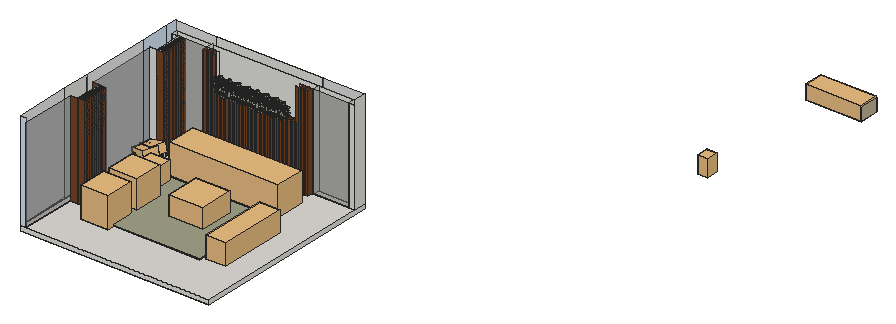
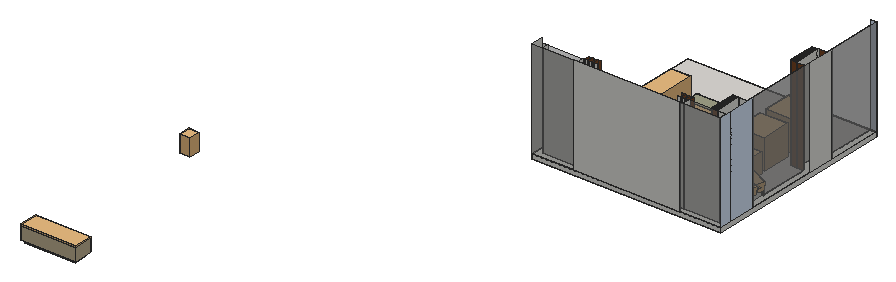
# SketchUp Ruby script. Lengths in inches.
U = 1.inch
M = Sketchup.active_model
def pt(a) = Geom::Point3d.new(a.map { |v| v * U })
def face(e, loops, mat)
  f = e.add_face(loops[0].map { |a| pt(a) })
  loops[1..].each { |l| e.add_face(l.map { |a| pt(a) }).erase! }
  f.material = f.back_material = mat if mat
  f
end
# faces: each face lists its corners as indices into pts; further lists are holes
def faces(e, pts, list, mat = nil) = list.each { |f| face(e, (f[0].is_a?(Array) ? f : [f]).map { |l| l.map { |i| pts[i] } }, mat) }
# xy, xz, yz: faces in a plane at the given z, y or x. An outline is a flat list of corners, or four numbers for a rectangle; further outlines are holes
def ring(l) = l.size == 4 ? [[l[0], l[1]], [l[2], l[1]], [l[2], l[3]], [l[0], l[3]]] : l.each_slice(2).to_a
def flat(e, list, mat, &to3) = list.each { |f| face(e, (f[0].is_a?(Array) ? f : [f]).map { |l| ring(l).map { |u, v| to3.(u, v) } }, mat) }
def xy(e, z, list, mat = nil) = flat(e, list, mat) { |x, y| [x, y, z] }
def xz(e, y, list, mat = nil) = flat(e, list, mat) { |x, z| [x, y, z] }
def yz(e, x, list, mat = nil) = flat(e, list, mat) { |y, z| [x, y, z] }
def lines(e, pts, list) = list.each { |a, b| e.add_line(pt(pts[a]), pt(pts[b])) }
# prism: a flat outline (further loops are holes) pulled along v
def prism(e, loops, v, mat = nil)
  f = face(e, loops, mat); d = Geom::Vector3d.new(v.map { |x| x * U })
  f.pushpull(f.normal.samedirection?(d) ? d.length : -d.length)
end
def box(e, o, s, mat = nil) = prism(e, [[o, [o[0] + s[0], o[1], o[2]], [o[0] + s[0], o[1] + s[1], o[2]], [o[0], o[1] + s[1], o[2]]]], [0, 0, s[2]], mat)
def at(x, y, z, deg = 0) = Geom::Transformation.translation(pt([x, y, z])) * Geom::Transformation.rotation(ORIGIN, Z_AXIS, deg.degrees)
def axes(o, x, y, z) = Geom::Transformation.new([*x, 0, *y, 0, *z, 0, *pt(o).to_a, 1])
def part(name) = M.definitions.add(name)
# library, detail: a bought-in or finely detailed component or shape, given as its bounding box
def library(name, o, s) = part(name).tap { |d| box(d.entities, o, s) }
def detail(e, o, s) = box(e.add_group.entities, o, s)
def put(e, d, t, mat = nil) = e.add_instance(d, t).tap { |i| i.material = mat if mat }
def group(e, t, mat = nil) = e.add_group.tap { |g| g.transformation = t; g.material = mat if mat }.entities
root = M.entities
M.materials.add("Generic").color = [214, 229, 247]
M.materials.add("Material__1").color = [190, 136, 85]
M.materials.add("Material__2").color = [51, 42, 44]
M.materials.add("Material__3").color = [119, 136, 107]
M.materials.add("Wood Fine AI 03").color = [193, 179, 148]
M.materials.add("Wood Fine AI 03-CW").color = [193, 179, 148]
M.materials.add("[0133_Gray]").color = [153, 153, 153]
M.materials.add("[Carpet Plush Forest]").color = [88, 100, 86]
M.materials.add("[Fabric Linen]").color = [161, 161, 136]
M.materials.add("[Terrazzo Tile Accent]").color = [221, 218, 214]
M.materials.add("[Translucent Glass Gray]").color = [128, 128, 128]
M.materials["[Translucent Glass Gray]"].alpha = 0.5
M.materials.add("[Wood Veneer 01]").color = [120, 70, 37]
M.materials.add("hymenocallis littoralis").color = [156, 172, 146]
c1 = library("_cadeira_03",[-17.72,-14.17,0],[35.44,28.34,38.23])
c2 = library("Lounge sofa",[0.125,0,0],[128.54,38.9,37.5625])
c3 = library("3dSolid\#17",[0,0,0],[103.74,27.56,5.91])
c4 = part("Group\#9")
xy(c4.entities,192,[[0,0,13.0625,3.375]])
xz(c4.entities,0,[[0,0,13.0625,192]])
xz(c4.entities,3.375,[[0,0,13.0625,192]])
yz(c4.entities,13.0625,[[0,0,3.375,192]])
c5 = part("Group\#1")
xy(c5.entities,18.5,[[0,0,1.625,2.0625]])
xz(c5.entities,0,[[0,0,1.625,18.5]])
xz(c5.entities,2.0625,[[0,0,1.625,18.5]])
yz(c5.entities,1.625,[[0,0,2.0625,18.5]])
c6 = part("Group\#10")
xy(c6.entities,18.5,[[0,0,1.6875,1.1875]])
xz(c6.entities,0,[[0,0,1.6875,18.5]])
yz(c6.entities,1.6875,[[0,0,1.1875,18.5]])
c7 = library("Group\#4",[0,0,0],[39.37,39.37,24.02])
c8 = library("Table3",[0,0,0],[60,20.45,30.02])
c9 = library("Group\#8",[0,0,0],[22.08,22.08,13.4])
c10 = part("DDR842RVS01100X")
xy(c10.entities,0,[[-70.87,0,47.24,78.74]])
xy(c10.entities,0.39,[[-70.87,0,47.24,78.74]],"[Fabric Linen]")
xz(c10.entities,0,[[-70.87,0,47.24,0.39]])
xz(c10.entities,78.74,[[-70.87,0,47.24,0.39]])
yz(c10.entities,-70.87,[[0,0,78.74,0.39]])
yz(c10.entities,47.24,[[0,0,78.74,0.39]])
c11 = part("Union")
xy(c11.entities,0,[[0,0,112.99,36.8125]],"Wood Fine AI 03-CW")
xy(c11.entities,1.38,[[1.38,0,111.61,35.43]],"Wood Fine AI 03-CW")
xy(c11.entities,25.59,[[0,0,1.38,0,1.38,35.43,0,36.8125],[111.61,0,112.99,0,112.99,36.8125,111.61,35.43]],"Wood Fine AI 03")
xy(c11.entities,25.59,[[1.38,35.43,111.61,35.43,112.99,36.8125,0,36.8125]],"Wood Fine AI 03-CW")
xz(c11.entities,0,[[0,0,1.38,1.38,1.38,25.59,0,25.59],[112.99,0,112.99,25.59,111.61,25.59,111.61,1.38]],"Wood Fine AI 03")
xz(c11.entities,0,[[0,0,112.99,0,111.61,1.38,1.38,1.38]],"Wood Fine AI 03-CW")
xz(c11.entities,35.43,[[1.38,1.38,111.61,25.59]],"Wood Fine AI 03")
xz(c11.entities,36.8125,[[0,0,112.99,25.59]],"Wood Fine AI 03")
yz(c11.entities,0,[[0,0,36.8125,25.59]],"Wood Fine AI 03")
yz(c11.entities,1.38,[[0,1.38,35.43,25.59]],"Wood Fine AI 03")
yz(c11.entities,111.61,[[0,1.38,35.43,25.59]],"Wood Fine AI 03")
yz(c11.entities,112.99,[[0,0,36.8125,25.59]],"Wood Fine AI 03")
c12 = library("Group\#6",[0,0,0],[111.61,37.58,26.77])
c13 = library("\#2",[-119.83,-119.83,113.8],[239.66,239.66,17.4])
c14 = library("\#4",[-204.92,-212.35,-236.71],[424.28,257.5,472.53])
c15 = part("\#3")
put(c15.entities,c14,axes([-0.37,309.72,0],[1.36765,0,0],[0,1.36765,0],[0,0,1.36765]),"Material__3")
c16 = library("\#1",[-174.07,-174.07,0],[348.14,348.14,140])
c17 = part("9")
put(c17.entities,c13,at(-19.94,-24.66,0),"Material__2")
put(c17.entities,c15,axes([17.67,-32.6,40.29],[0.29694,0.9549,0],[-0.21403,0.06656,0.97456],[0.9306,-0.28939,0.22414]))
put(c17.entities,c16,at(-19.94,-24.66,0),"Material__1")
c18 = library("Group",[-10.56,-10.46,-0.01],[21.3,22.85,34.81])
c19 = part("Group\#856")
xy(c19.entities,7.38,[[0,0,5.5,15.91]],"hymenocallis littoralis")
p = [[5.5,28.78,0],[5.5,26.79,3.44],[0,26.79,3.44],[0,28.78,0],[0,23.75,6],[5.5,23.75,6],
  [0,15.91,7.38],[5.5,15.91,7.38]]
faces(c19.entities,p,[[0,1,2,3],[4,2,1,5],[6,4,5,7]],"hymenocallis littoralis")
c20 = part("Group\#854")
xy(c20.entities,7.38,[[0,0,5.5,15.91],[0,15.91,5.5,23.87]],"hymenocallis littoralis")
p = [[5.5,31.07,4.3],[5.5,27.74,6.47],[0,27.74,6.47],[0,31.07,4.3],[0,23.87,7.38],[5.5,23.87,7.38]]
faces(c20.entities,p,[[0,1,2,3],[4,2,1,5]],"hymenocallis littoralis")
c21 = part("Group\#857")
xy(c21.entities,7.38,[[0,0,5.6,15.91]],"hymenocallis littoralis")
p = [[5.6,28.78,0],[5.6,26.79,3.44],[0,26.79,3.44],[0,28.78,0],[0,23.75,6],[5.6,23.75,6],
  [0,15.91,7.38],[5.6,15.91,7.38]]
faces(c21.entities,p,[[0,1,2,3],[4,2,1,5],[6,4,5,7]],"hymenocallis littoralis")
c22 = part("Group\#855")
put(c22.entities,c20,axes([6.09,8.57,-0.52],[0.446,0.85617,0.26089],[-0.18444,-0.19731,0.96283],[0.87582,-0.47754,0.0699]))
put(c22.entities,c20,axes([6.29,7.28,-1.71],[0.37058,0.92707,-0.05667],[-0.32382,0.19004,0.99128],[0.87712,-0.32925,0.34964]))
put(c22.entities,c20,axes([11.04,16.14,-0.7],[1,0,0],[0,0.16628,1.02662],[0,-1.18456,0.19186]))
c23 = part("Group\#860")
put(c23.entities,c19,axes([24.57,32.05,-1.76],[0.9552,-0.22102,-0.19681],[0.4036,0.95545,0.88585],[-0.00568,-0.67859,0.7345]))
put(c23.entities,c19,axes([23.95,29.24,-2.4],[0,1,0],[-0.76041,0,0.64945],[0.64945,0,0.76041]))
put(c23.entities,c19,axes([24.22,24.72,-0.48],[-0.70711,0.70711,0],[-0.32757,-0.32757,0.80237],[0.61237,0.61237,0.5]))
put(c23.entities,c20,axes([20.66,37.22,-0.63],[1.12361,0.03262,0.39091],[-0.43499,0.29739,0.78777],[0.09852,-1.27434,0.37535]))
put(c23.entities,c19,axes([28.75,24.45,-2.4],[-1,0,0],[0,-0.76041,0.64945],[0,0.64945,0.76041]))
put(c23.entities,c21,axes([30.4,30.98,-3.7],[0.65676,-0.72002,0.22414],[0.55667,0.66341,0.5],[-0.50871,-0.20361,0.83652]))
put(c23.entities,c21,axes([32.41,29.61,-3.7],[0.04029,-0.97372,0.22414],[0.85287,0.15038,0.5],[-0.52057,0.17102,0.83652]))
put(c23.entities,c19,axes([31.89,25.85,-1.76],[-0.92056,0.33739,-0.19681],[-0.5186,-0.89824,0.88585],[0.08952,0.67268,0.7345]))
put(c23.entities,c19,axes([25.55,34.78,-0.48],[0.86603,0.5,0],[-0.25,0.43301,0.86603],[0.43301,-0.75,0.5]))
put(c23.entities,c21,axes([20.4,16.9375,-8.07],[-0.70711,0.70711,0],[-0.35754,-0.35754,0.65422],[1.3987,1.3987,1.52882]))
put(c23.entities,c19,axes([32.86,34.14,-0.48],[0.76604,-0.64279,0],[0.32139,0.38302,0.86603],[-0.55667,-0.66341,0.5]))
put(c23.entities,c19,axes([27.15,34.7,-0.1],[0.82472,-0.17528,-0.53769],[0.53769,0.53769,0.64945],[0.17528,-0.82472,0.53769]))
put(c23.entities,c19,axes([33.58,28.77,-2.4],[0,-1,0],[0.76041,0,0.64945],[-0.64945,0,0.76041]))
put(c23.entities,c19,axes([26.43,23.87,-2.81],[-0.75126,0.04415,0.65853],[0.53769,-0.53769,0.64945],[0.38276,0.84199,0.3802]))
put(c23.entities,c19,axes([28.78,23.98,-2.4],[-1,0,0],[0,-0.76041,0.64945],[0,0.64945,0.76041]))
put(c23.entities,c19,axes([25.39,25.38,-2.4],[-0.70711,0.70711,0],[-0.53769,-0.53769,0.64945],[0.45923,0.45923,0.76041]))
put(c23.entities,c19,axes([27.32,21.63,-0.1],[-0.45923,0.70711,-0.53769],[-0.76041,0,0.64945],[0.45923,0.70711,0.53769]))
put(c23.entities,c19,axes([25.17,27.625,-1.76],[0.56416,0.80187,-0.19681],[-0.66673,0.66673,0.80532],[0.62659,-0.26057,0.7345]))
put(c23.entities,c21,axes([27.59,27.04,-3.96],[-0.8993,-0.06127,0.43301],[0.2962,-0.8138,0.5],[0.32175,0.57791,0.75]))
put(c23.entities,c21,axes([26.98,24.5,-3.18],[-0.5,0.86603,0],[-0.75,-0.43301,0.5],[0.43301,0.25,0.86603]))
put(c23.entities,c21,axes([24.55,27.74,-3.7],[0.29517,0.92878,0.22414],[-0.85287,0.15038,0.5],[0.43068,-0.33875,0.83652]))
put(c23.entities,c21,axes([24.26,29.8,-3.18],[0.76604,0.64279,0],[-0.47317,0.5639,0.425],[0.32139,-0.38302,0.86603]))
put(c23.entities,c21,axes([25.98,32.46,-3.18],[1,0,0],[0,0.86603,0.5],[0,-0.5,0.86603]))
put(c23.entities,c19,axes([28.78,33.57,-2.4],[1,0,0],[0,0.76041,0.64945],[0,-0.64945,0.76041]))
put(c23.entities,c22,at(14.99,21.38,2.5))
put(c23.entities,c20,axes([34.63,26.34,-1.46],[-0.70089,-0.70877,0.07994],[0.4756,-0.38088,0.79293],[-0.53156,0.59378,0.60405]))
put(c23.entities,c20,axes([28.14,16.92,1.8125],[-1.19719,0.6912,0],[-0.09607,-0.16641,0.94244],[0.68444,1.18549,0.17613]))
put(c23.entities,c20,axes([31.5625,35.84,0.97],[0.66765,-1.1564,0.35779],[0.04445,0.30732,0.91033],[-1.20828,-0.64496,0.17012]))
put(c23.entities,c20,axes([38.94,22.51,0.89],[-0.97932,-0.67164,-0.05202],[0.27787,-0.41401,0.90999],[-0.85985,0.93577,0.32097]))
put(c23.entities,c20,axes([38.44,21.09,1.98],[-1.02864,-0.54856,0.2395],[0.33481,0.06999,0.88388],[-0.77261,1.08328,0.06417]))
put(c23.entities,c21,axes([35.02,30.51,-1.3],[-0.17365,-0.98481,0],[0.60224,-0.10619,0.79122],[-0.7792,0.13739,0.61153]))
put(c23.entities,c21,axes([29.41,22.33,-1.3],[-0.93969,0.34202,0],[-0.20915,-0.57465,0.79122],[0.27061,0.74351,0.61153]))
put(c23.entities,c20,axes([19.64,36,-1.62],[1.18194,0.09546,0.08234],[-0.14377,0.68823,0.76313],[0.21457,-1.1326,0.62386]))
put(c23.entities,c21,axes([24.25,24.14,-1.3],[-0.34202,0.93969,0],[-0.57465,-0.20915,0.79122],[0.74351,0.27061,0.61153]))
put(c23.entities,c21,axes([25.98,34.61,-1.3],[1,0,0],[0,0.61153,0.79122],[0,-0.79122,0.61153]))
put(c23.entities,c21,axes([31.16,34.41,-1.64],[0.56518,-0.80224,-0.19234],[0.73413,0.34233,0.72935],[-0.47639,-0.50772,0.71782]))
put(c23.entities,c21,axes([40.52,26.84,-5.82],[-0.42262,-0.90631,0],[0.48019,-0.22391,0.68552],[-1.43418,0.66877,1.22305]))
put(c23.entities,c19,axes([29.86,38.42,-1.01],[0.89064,-0.37013,0.26413],[-0.03924,0.63286,1.01918],[-0.45353,-0.76487,0.45748]))
put(c23.entities,c19,axes([29.34,22.4,-0.48],[-0.99619,-0.08716,0],[0.04358,-0.4981,0.86603],[-0.07548,0.86273,0.5]))
c24 = part("Group\#858")
xz(c24.entities,10.07,[[9.07,0,10.07,31.01],[0,31.01,0,45.12,20.13,45.12,20.13,31.01,10.07,31.01,10.07,32.58,9.07,32.58,9.07,31.01]],"hymenocallis littoralis")
yz(c24.entities,10.07,[[0,31.01,20.13,45.12]],"hymenocallis littoralis")
p = [[9.57,9.2,0],[10.07,10.07,0],[10.07,10.07,31.01],[10.07,10.07,32.58],[9.57,9.2,32.58]]
faces(c24.entities,p,[[0,1,2,3,4]],"hymenocallis littoralis")
c25 = part("cây lá nắng")
put(c25.entities,c23,axes([49.26,-2.75,0],[0.63109,0.63109,0],[-0.63109,0.63109,0],[0,0,0.935]))
g1 = group(c25.entities,at(26.6,-8.68,0))
put(g1,c19,axes([-4.72,35.73,-1.65],[0.74231,0.46334,-0.18402],[-0.34827,0.85768,0.82827],[0.42467,-0.43184,0.68675]))
put(g1,c19,axes([-3.34,33.57,-2.24],[-0.63109,0.63109,0],[-0.47989,-0.47989,0.60723],[0.40986,0.40986,0.71098]))
put(g1,c19,axes([-0.3125,30.89,-0.45],[-0.8925,0,0],[0,-0.41345,0.75022],[0,0.77293,0.4675]))
put(g1,c20,axes([-10.79,39.66,-0.59],[0.68852,0.72969,0.3655],[-0.4622,-0.08684,0.73657],[0.86641,-0.74205,0.35095]))
put(g1,c19,axes([2.71,33.57,-2.24],[-0.63109,-0.63109,0],[0.47989,-0.47989,0.60723],[-0.40986,0.40986,0.71098]))
put(g1,c21,axes([-0.37,38.74,-3.46],[0.86887,-0.03992,0.20957],[-0.06737,0.76999,0.4675],[-0.19255,-0.44954,0.78214]))
put(g1,c21,axes([1.76,39.14,-3.46],[0.63993,-0.58908,0.20957],[0.44333,0.63315,0.4675],[-0.43646,-0.2206,0.78214]))
put(g1,c19,axes([3.81,36.4375,-1.65],[-0.79389,-0.36803,-0.18402],[0.23959,-0.89415,0.82827],[-0.36803,0.48102,0.68675]))
put(g1,c19,axes([-5.83,38.07,-0.45],[0.231,0.86209,0],[-0.43104,0.1155,0.80973],[0.74659,-0.20005,0.4675]))
put(g1,c21,axes([2.18,23.5625,-7.55],[-0.8925,0,0],[0,-0.45128,0.6117],[0,1.76542,1.42944]))
put(g1,c19,axes([-0.8125,42.28,-0.45],[0.8891,0.07779,0],[-0.03889,0.44455,0.80973],[0.06737,-0.76999,0.4675]))
put(g1,c19,axes([-4.76,39.03,-0.09],[0.63109,0.40986,-0.50274],[0,0.67866,0.60723],[0.63109,-0.40986,0.50274]))
put(g1,c19,axes([3.03,39.35,-2.24],[0.63109,-0.63109,0],[0.47989,0.47989,0.60723],[-0.40986,-0.40986,0.71098]))
put(g1,c19,axes([1.61,31.74,-2.625],[-0.50198,-0.44625,0.61573],[0.67866,0,0.60723],[-0.28982,0.77293,0.35549]))
put(g1,c19,axes([3.03,33.3,-2.24],[-0.63109,-0.63109,0],[0.47989,-0.47989,0.60723],[-0.40986,0.40986,0.71098]))
put(g1,c19,axes([0.01,32.04,-2.24],[-0.8925,0,0],[0,-0.67866,0.60723],[0,0.57963,0.71098]))
put(g1,c19,axes([3.59,30.89,-0.09],[-0.73607,0.15643,-0.50274],[-0.47989,-0.47989,0.60723],[-0.15643,0.73607,0.50274]))
put(g1,c19,axes([-1.55,33.32,-1.65],[-0.15002,0.86209,-0.18402],[-0.84154,0,0.75297],[0.55988,0.231,0.68675]))
put(g1,c21,axes([0.35,34.48,-3.71],[-0.52887,-0.60621,0.40487],[0.70051,-0.32665,0.4675],[-0.16166,0.56777,0.70125]))
put(g1,c21,axes([2.61,39.13,-1.74],[-0.86209,0.231,0],[-0.23031,-0.85954,0.15531],[0.03162,0.11799,0.91645]))
put(g1,c21,axes([-2.02,33,-3.46],[-0.39986,0.77243,0.20957],[-0.63315,-0.44333,0.4675],[0.48558,0.05802,0.78214]))
put(g1,c21,axes([-3.49,34.12,-2.97],[0.07779,0.8891,0],[-0.65449,0.05726,0.39737],[0.44455,-0.03889,0.80973]))
put(g1,c21,axes([-4.09,36.88,-2.97],[0.63109,0.63109,0],[-0.54654,0.54654,0.4675],[0.31555,-0.31555,0.80973]))
put(g1,c19,axes([-3.02,39.35,-2.24],[0.63109,0.63109,0],[-0.47989,0.47989,0.60723],[0.40986,-0.40986,0.71098]))
put(g1,c22,axes([-4.03,22.95,2.33],[0.63109,0.63109,0],[-0.63109,0.63109,0],[0,0,0.935]))
put(g1,c20,axes([5.24,38.48,-1.37],[0.00497,-0.88963,0.07474],[0.54052,0.05978,0.74139],[-0.71019,0.03927,0.56479]))
put(g1,c20,axes([7.08,28.4375,1.7],[-1.19175,-0.31933,0],[0.04439,-0.16565,0.88118],[-0.31621,1.1801,0.16468]))
put(g1,c20,axes([-2.7,42.54,0.91],[1.15114,-0.30845,0.33454],[-0.1659,0.22199,0.85115],[-0.3555,-1.16957,0.15907]))
put(g1,c20,axes([10.37,38.78,0.83],[-0.19417,-1.04191,-0.04864],[0.43664,-0.08592,0.85084],[-1.1332,0.04791,0.30011]))
put(g1,c20,axes([10.95,37.5625,1.85],[-0.30298,-0.99536,0.22393],[0.16713,0.25547,0.82643],[-1.17124,0.19607,0.06]))
put(g1,c21,axes([2.84,41.36,-1.22],[0.51192,-0.73109,0],[0.44708,0.31305,0.73979],[-0.57846,-0.40504,0.57178]))
put(g1,c21,axes([4.47,32.65,-1.22],[-0.80888,-0.37719,0],[0.23066,-0.49465,0.73979],[-0.29844,0.64,0.57178]))
put(g1,c20,axes([-10.32,35.12,-1.51],[0.68567,0.80616,0.07699],[-0.52507,0.3436,0.71352],[0.85019,-0.57936,0.58331]))
put(g1,c21,axes([0.07,30.54,-1.22],[-0.80888,0.37719,0],[-0.23066,-0.49465,0.73979],[0.29844,0.64,0.57178]))
put(g1,c21,axes([-5.45,38.24,-1.22],[0.63109,0.63109,0],[-0.38593,0.38593,0.73979],[0.49934,-0.49934,0.57178]))
put(g1,c21,axes([-2.05,41.38,-1.53],[0.86296,-0.14961,-0.17984],[0.24726,0.67935,0.68194],[0.01977,-0.62107,0.67116]))
put(g1,c21,axes([8.63,42.51,-5.4375],[0.30525,-0.83868,0],[0.44435,0.16173,0.64096],[-1.32716,-0.48305,1.14356]))
put(g1,c19,axes([-5.4,43.09,-0.94],[0.79566,0.32849,0.24696],[-0.42416,0.37462,0.95293],[0.19648,-0.76892,0.42774]))
put(g1,c19,axes([4.38,32.65,-0.45],[-0.57369,-0.68369,0],[0.34185,-0.28684,0.80973],[-0.5921,0.49683,0.4675]))
put(g1,c21,axes([-2,33.84,-0.15],[-0.24601,0.85793,0],[-0.85539,-0.24528,0.15531],[0.11742,0.03367,0.91645]))
put(g1,c21,axes([0.17,30.83,-4.47],[-0.24601,0.85793,0],[-0.85539,-0.24528,0.15531],[0.11742,0.03367,0.91645]))
put(g1,c21,axes([-1.97,32.18,-4.47],[0.58524,0.67383,0],[-0.67184,0.58351,0.15531],[0.09222,-0.0801,0.91645]))
put(g1,c21,axes([-2,34.71,-4.47],[0.88392,-0.12346,0],[0.12309,0.88131,0.15531],[-0.0169,-0.12098,0.91645]))
put(g1,c21,axes([0.11,36.12,-4.47],[0.37822,-0.8084,0],[0.80601,0.37711,0.15531],[-0.11064,-0.05177,0.91645]))
put(c25.entities,c24,axes([29.71,14.29,6.94],[0.425,0.73612,0],[-0.6771,0.39092,-0.33349],[-0.26859,0.15507,0.72712]))
put(c25.entities,c24,axes([42.0625,26.12,6.94],[0.85,0,0],[0,0.78185,-0.33349],[0,0.33349,0.78185]))
put(c25.entities,c23,axes([7.3125,23.0625,0],[0.8925,0,0],[0,0.8925,0],[0,0,0.935]))
put(c25.entities,c24,axes([24.4375,40.23,2.05],[0.85,0,0],[0,0.85,0],[0,0,0.85]))
c26 = part("Planting+101")
put(c26.entities,c25,axes([21.34,32.96,-4.59],[0,-0.71,0],[-0.71,0,0],[0,0,0.71]))
xy(root,-9,[[0,0,384,396]])
xy(root,-0.625,[[15.09,275.22,36.97,311.16]])
xy(root,0,[[0,0,12,0,12,113.46,27,113.46,27,168.59,12,168.59,12,272.125,27,272.125,27,370.9375,12,370.9375,12,384,372,384,372,370.9375,384,370.9375,384,396,0,396],[27,113.46,40.0625,116.84],[12,270.9375,13.6875,272.125],[40.0625,272.125,41.6875,274.1875],[84,360.5625,90.4375,370.9375],
  [12,370.9375,84,384],[84,370.9375,300,384],[300,370.9375,372,384]])
xy(root,0,[[12,0,384,0,384,370.9375,297.4375,370.9375,297.4375,360.5625,291,360.5625,291,370.9375,288.4375,370.9375,288.4375,360.5625,282,360.5625,282,370.9375,279.4375,370.9375,279.4375,360.5625,273,360.5625,273,370.9375,270.4375,370.9375,270.4375,360.5625,264,360.5625,264,370.9375,261.4375,370.9375,261.4375,360.5625,255,360.5625,255,370.9375,252.4375,370.9375,252.4375,360.5625,246,360.5625,246,370.9375,243.4375,370.9375,243.4375,360.5625,237,360.5625,237,370.9375,234.4375,370.9375,234.4375,360.5625,228,360.5625,228,370.9375,225.4375,370.9375,225.4375,360.5625,219,360.5625,219,370.9375,216.4375,370.9375,216.4375,360.5625,210,360.5625,210,370.9375,207.4375,370.9375,207.4375,360.5625,201,360.5625,201,370.9375,198.4375,370.9375,198.4375,360.5625,192,360.5625,192,370.9375,189.4375,370.9375,189.4375,360.5625,183,360.5625,183,370.9375,180.4375,370.9375,180.4375,360.5625,174,360.5625,174,370.9375,171.4375,370.9375,171.4375,360.5625,165,360.5625,165,370.9375,162.4375,370.9375,162.4375,360.5625,156,360.5625,156,370.9375,153.4375,370.9375,153.4375,360.5625,147,360.5625,147,370.9375,144.4375,370.9375,144.4375,360.5625,138,360.5625,138,370.9375,135.4375,370.9375,135.4375,360.5625,129,360.5625,129,370.9375,126.4375,370.9375,126.4375,360.5625,120,360.5625,120,370.9375,117.4375,370.9375,117.4375,360.5625,111,360.5625,111,370.9375,108.4375,370.9375,108.4375,360.5625,102,360.5625,102,370.9375,99.4375,370.9375,99.4375,360.5625,93,360.5625,93,370.9375,90.4375,370.9375,90.4375,360.5625,84,360.5625,84,370.9375,27,370.9375,27,317.625,40.0625,317.625,40.0625,274.1875,41.6875,274.1875,41.6875,272.125,13.6875,272.125,13.6875,270.9375,12,270.9375,12,168.59,27,168.59,27,116.84,40.0625,116.84,40.0625,113.46,12,113.46],[27,272.125,40.0625,317.625],[93,360.5625,99.4375,370.9375],[102,360.5625,108.4375,370.9375],[111,360.5625,117.4375,370.9375],
  [120,360.5625,126.4375,370.9375],[129,360.5625,135.4375,370.9375],[138,360.5625,144.4375,370.9375],[147,360.5625,153.4375,370.9375],[156,360.5625,162.4375,370.9375],
  [165,360.5625,171.4375,370.9375],[174,360.5625,180.4375,370.9375],[183,360.5625,189.4375,370.9375],[192,360.5625,198.4375,370.9375],[201,360.5625,207.4375,370.9375],
  [210,360.5625,216.4375,370.9375],[219,360.5625,225.4375,370.9375],[228,360.5625,234.4375,370.9375],[237,360.5625,243.4375,370.9375],[246,360.5625,252.4375,370.9375],
  [255,360.5625,261.4375,370.9375],[264,360.5625,270.4375,370.9375],[273,360.5625,279.4375,370.9375],[282,360.5625,288.4375,370.9375],[291,360.5625,297.4375,370.9375]],"[Terrazzo Tile Accent]")
xy(root,18.5,[[[12,272.125,40.0625,314.25],[15.09,275.22,36.97,311.16]]])
xz(root,0,[[0,-9,384,0]])
xz(root,0,[[0,0,12,200.8125]],"Generic")
xz(root,113.46,[[12,0,27,192]],"[Wood Veneer 01]")
xz(root,168.59,[[12,0,27,192]],"[Wood Veneer 01]")
xz(root,272.125,[[12,0,13.6875,18.5],[13.6875,0,40.0625,18.5]])
xz(root,275.22,[[15.09,-0.625,36.97,18.5]])
xz(root,311.16,[[15.09,-0.625,27,18.5],[27,-0.625,36.97,18.5]])
xz(root,314.25,[[12,18.5,27,192]])
xz(root,314.25,[[27,18.5,40.0625,192]],"[Wood Veneer 01]")
xz(root,317.625,[[27,0,40.0625,192]])
xz(root,360.5625,[[84,0,90.4375,192],[93,0,99.4375,192],[102,0,108.4375,192],[111,0,117.4375,125.75],[120,0,126.4375,125.75],
  [129,0,135.4375,125.75],[138,0,144.4375,125.75],[147,0,153.4375,125.75],[156,0,162.4375,125.75],[165,0,171.4375,125.75],
  [174,0,180.4375,125.75],[183,0,189.4375,125.75],[192,0,198.4375,125.75],[201,0,207.4375,125.75],[210,0,216.4375,125.75],
  [219,0,225.4375,125.75],[228,0,234.4375,125.75],[237,0,243.4375,125.75],[246,0,252.4375,125.75],[255,0,261.4375,125.75],
  [264,0,270.4375,125.75],[273,0,279.4375,192],[282,0,288.4375,192],[291,0,297.4375,192]],"[Wood Veneer 01]")
xz(root,370.9375,[[12,0,27,192],[84,0,90.4375,192],[90.4375,0,93,192],[93,0,99.4375,192],[99.4375,0,102,192],
  [102,0,108.4375,192],[108.4375,0,111,125.75],[111,0,117.4375,125.75],[117.4375,0,120,125.75],[120,0,126.4375,125.75],
  [126.4375,0,129,125.75],[129,0,135.4375,125.75],[135.4375,0,138,125.75],[138,0,144.4375,125.75],[144.4375,0,147,125.75],
  [147,0,153.4375,125.75],[153.4375,0,156,125.75],[156,0,162.4375,125.75],[162.4375,0,165,125.75],[165,0,171.4375,125.75],
  [171.4375,0,174,125.75],[174,0,180.4375,125.75],[180.4375,0,183,125.75],[183,0,189.4375,125.75],[189.4375,0,192,125.75],
  [192,0,198.4375,125.75],[198.4375,0,201,125.75],[201,0,207.4375,125.75],[207.4375,0,210,125.75],[210,0,216.4375,125.75],
  [216.4375,0,219,125.75],[219,0,225.4375,125.75],[225.4375,0,228,125.75],[228,0,234.4375,125.75],[234.4375,0,237,125.75],
  [237,0,243.4375,125.75],[243.4375,0,246,125.75],[246,0,252.4375,125.75],[252.4375,0,255,125.75],[255,0,261.4375,125.75],
  [261.4375,0,264,125.75],[264,0,270.4375,125.75],[270.4375,0,273,125.75],[273,0,279.4375,192],[279.4375,0,282,192],
  [282,0,288.4375,192],[288.4375,0,291,192],[291,0,297.4375,192],[372,0,384,191.375]])
xz(root,370.9375,[[27,0,84,192],[300,0,372,192]],"[Translucent Glass Gray]")
xz(root,370.9375,[[297.4375,0,300,192]],"[Wood Veneer 01]")
xz(root,384,[[12,0,84,191.375],[84,0,300,191.375],[300,0,372,191.375]])
xz(root,396,[[0,-9,384,0],[84,0,300,200.8125]])
xz(root,396,[[0,0,84,200.8125],[300,0,384,200.8125]],"[Translucent Glass Gray]")
yz(root,0,[[0,-9,396,0],[113.46,0,170.15,200.8125]])
yz(root,0,[[314.25,0,370.9375,200.8125],[370.9375,0,396,200.8125]],"Generic")
yz(root,0,[[0,0,113.46,200.8125],[170.15,0,314.25,200.8125]],"[Translucent Glass Gray]")
yz(root,12,[[270.9375,0,272.125,18.5],[370.9375,0,384,191.375]])
yz(root,12,[[0,0,113.46,191.375],[168.59,0,270.9375,0,270.9375,18.5,314.25,18.5,314.25,191.375,168.59,191.375]],"[Translucent Glass Gray]")
yz(root,15.09,[[275.22,-0.625,311.16,18.5]])
yz(root,27,[[113.46,0,116.84,192],[116.84,0,168.59,192],[317.625,0,370.9375,192]])
yz(root,36.97,[[275.22,-0.625,311.16,18.5]])
yz(root,40.0625,[[272.125,0,274.1875,18.5]])
yz(root,40.0625,[[274.1875,0,317.625,0,317.625,192,314.25,192,314.25,18.5,274.1875,18.5]],"[Wood Veneer 01]")
yz(root,84,[[370.9375,0,384,192]])
yz(root,84,[[360.5625,0,370.9375,192]],"[Wood Veneer 01]")
yz(root,90.4375,[[360.5625,0,370.9375,192]],"[Wood Veneer 01]")
yz(root,93,[[360.5625,0,370.9375,192]],"[Wood Veneer 01]")
yz(root,99.4375,[[360.5625,0,370.9375,192]],"[Wood Veneer 01]")
yz(root,102,[[360.5625,0,370.9375,192]],"[Wood Veneer 01]")
yz(root,108.4375,[[360.5625,0,370.9375,125.75]],"[Wood Veneer 01]")
yz(root,111,[[360.5625,0,370.9375,125.75]],"[Wood Veneer 01]")
yz(root,117.4375,[[360.5625,0,370.9375,125.75]],"[Wood Veneer 01]")
yz(root,120,[[360.5625,0,370.9375,125.75]],"[Wood Veneer 01]")
yz(root,126.4375,[[360.5625,0,370.9375,125.75]],"[Wood Veneer 01]")
yz(root,129,[[360.5625,0,370.9375,125.75]],"[Wood Veneer 01]")
yz(root,135.4375,[[360.5625,0,370.9375,125.75]],"[Wood Veneer 01]")
yz(root,138,[[360.5625,0,370.9375,125.75]],"[Wood Veneer 01]")
yz(root,144.4375,[[360.5625,0,370.9375,125.75]],"[Wood Veneer 01]")
yz(root,147,[[360.5625,0,370.9375,125.75]],"[Wood Veneer 01]")
yz(root,153.4375,[[360.5625,0,370.9375,125.75]],"[Wood Veneer 01]")
yz(root,156,[[360.5625,0,370.9375,125.75]],"[Wood Veneer 01]")
yz(root,162.4375,[[360.5625,0,370.9375,125.75]],"[Wood Veneer 01]")
yz(root,165,[[360.5625,0,370.9375,125.75]],"[Wood Veneer 01]")
yz(root,171.4375,[[360.5625,0,370.9375,125.75]],"[Wood Veneer 01]")
yz(root,174,[[360.5625,0,370.9375,125.75]],"[Wood Veneer 01]")
yz(root,180.4375,[[360.5625,0,370.9375,125.75]],"[Wood Veneer 01]")
yz(root,183,[[360.5625,0,370.9375,125.75]],"[Wood Veneer 01]")
yz(root,189.4375,[[360.5625,0,370.9375,125.75]],"[Wood Veneer 01]")
yz(root,192,[[360.5625,0,370.9375,125.75]],"[Wood Veneer 01]")
yz(root,198.4375,[[360.5625,0,370.9375,125.75]],"[Wood Veneer 01]")
yz(root,201,[[360.5625,0,370.9375,125.75]],"[Wood Veneer 01]")
yz(root,207.4375,[[360.5625,0,370.9375,125.75]],"[Wood Veneer 01]")
yz(root,210,[[360.5625,0,370.9375,125.75]],"[Wood Veneer 01]")
yz(root,216.4375,[[360.5625,0,370.9375,125.75]],"[Wood Veneer 01]")
yz(root,219,[[360.5625,0,370.9375,125.75]],"[Wood Veneer 01]")
yz(root,225.4375,[[360.5625,0,370.9375,125.75]],"[Wood Veneer 01]")
yz(root,228,[[360.5625,0,370.9375,125.75]],"[Wood Veneer 01]")
yz(root,234.4375,[[360.5625,0,370.9375,125.75]],"[Wood Veneer 01]")
yz(root,237,[[360.5625,0,370.9375,125.75]],"[Wood Veneer 01]")
yz(root,243.4375,[[360.5625,0,370.9375,125.75]],"[Wood Veneer 01]")
yz(root,246,[[360.5625,0,370.9375,125.75]],"[Wood Veneer 01]")
yz(root,252.4375,[[360.5625,0,370.9375,125.75]],"[Wood Veneer 01]")
yz(root,255,[[360.5625,0,370.9375,125.75]],"[Wood Veneer 01]")
yz(root,261.4375,[[360.5625,0,370.9375,125.75]],"[Wood Veneer 01]")
yz(root,264,[[360.5625,0,370.9375,125.75]],"[Wood Veneer 01]")
yz(root,270.4375,[[360.5625,0,370.9375,125.75]],"[Wood Veneer 01]")
yz(root,273,[[360.5625,0,370.9375,125.75]],"[Wood Veneer 01]")
yz(root,279.4375,[[360.5625,0,370.9375,192]],"[Wood Veneer 01]")
yz(root,282,[[360.5625,0,370.9375,192]],"[Wood Veneer 01]")
yz(root,288.4375,[[360.5625,0,370.9375,192]],"[Wood Veneer 01]")
yz(root,291,[[360.5625,0,370.9375,192]],"[Wood Veneer 01]")
yz(root,297.4375,[[360.5625,0,370.9375,192]],"[Wood Veneer 01]")
yz(root,300,[[370.9375,0,384,192]])
yz(root,372,[[370.9375,0,384,191.375]])
yz(root,384,[[0,-9,396,0],[370.9375,0,396,200.8125]])
put(root,c1,axes([88.52,179.09,0],[1.5972,0,0],[0,2.07636,0],[0,0,1.5972]))
put(root,c1,axes([88.52,107.09,0],[1.5972,0,0],[0,2.07636,0],[0,0,1.5972]))
put(root,c2,axes([80.63,276.04,0],[1.73652,0,0],[0,1.57865,0],[0,0,1.57865]))
put(root,c3,at(730.28,1098.67,0))
put(root,c4,at(27,113.46,0),"[Wood Veneer 01]")
put(root,c4,at(27,117.77,0),"[Wood Veneer 01]")
put(root,c4,at(27,122.09,0),"[Wood Veneer 01]")
put(root,c4,at(27,126.4,0),"[Wood Veneer 01]")
put(root,c4,at(27,130.71,0),"[Wood Veneer 01]")
put(root,c4,at(27,135.02,0),"[Wood Veneer 01]")
put(root,c4,at(27,139.34,0),"[Wood Veneer 01]")
put(root,c4,at(27,143.65,0),"[Wood Veneer 01]")
put(root,c4,at(27,147.96,0),"[Wood Veneer 01]")
put(root,c4,at(27,152.27,0),"[Wood Veneer 01]")
put(root,c4,at(27,156.59,0),"[Wood Veneer 01]")
put(root,c4,at(27,160.9,0),"[Wood Veneer 01]")
put(root,c4,at(27,165.21,0),"[Wood Veneer 01]")
put(root,c4,at(27,331.5,0),"[Wood Veneer 01]")
put(root,c4,at(27,335.8125,0),"[Wood Veneer 01]")
put(root,c4,at(27,327.1875,0),"[Wood Veneer 01]")
put(root,c4,at(27,340.125,0),"[Wood Veneer 01]")
put(root,c4,at(27,348.75,0),"[Wood Veneer 01]")
put(root,c4,at(27,322.875,0),"[Wood Veneer 01]")
put(root,c4,at(27,344.4375,0),"[Wood Veneer 01]")
put(root,c4,at(27,353.0625,0),"[Wood Veneer 01]")
put(root,c4,at(27,357.375,0),"[Wood Veneer 01]")
put(root,c4,at(27,361.6875,0),"[Wood Veneer 01]")
put(root,c4,at(27,366,0),"[Wood Veneer 01]")
put(root,c4,at(27,318.5625,0),"[Wood Veneer 01]")
put(root,c5,at(40.0625,272.125,0))
put(root,c5,at(40.0625,274.8125,0))
put(root,c5,at(40.0625,277.5,0))
put(root,c5,at(40.0625,280.1875,0))
put(root,c5,at(40.0625,282.875,0))
put(root,c5,at(40.0625,285.5625,0))
put(root,c5,at(40.0625,288.25,0))
put(root,c5,at(40.0625,290.9375,0))
put(root,c5,at(40.0625,293.625,0))
put(root,c5,at(40.0625,296.3125,0))
put(root,c5,at(40.0625,299,0))
put(root,c5,at(40.0625,301.6875,0))
put(root,c5,at(40.0625,304.375,0))
put(root,c5,at(40.0625,307.0625,0))
put(root,c5,at(40.0625,309.75,0))
put(root,c5,at(40.0625,312.4375,0))
put(root,c6,at(12,270.9375,0))
put(root,c6,at(14.125,270.9375,0))
put(root,c6,at(16.25,270.9375,0))
put(root,c6,at(18.375,270.9375,0))
put(root,c6,at(20.5,270.9375,0))
put(root,c6,at(22.625,270.9375,0))
put(root,c6,at(24.75,270.9375,0))
put(root,c6,at(26.875,270.9375,0))
put(root,c6,at(29,270.9375,0))
put(root,c6,at(31.125,270.9375,0))
put(root,c6,at(33.25,270.9375,0))
put(root,c6,at(35.375,270.9375,0))
put(root,c6,at(37.5,270.9375,0))
put(root,c6,at(39.625,270.9375,0))
put(root,c7,axes([58.5,218.82,0],[1,0,0],[0,1,0],[0,0,1.69]))
put(root,c8,axes([296.68,238.52,0],[0,-2.2946,0],[2,0,0],[0,0,1.41]))
put(root,c9,axes([168.1,166.73,0],[3.1598,0,0],[0,3.1598,0],[0,0,3.1598]))
put(root,c10,axes([209.68,86.22,3.86],[1.82,0,0],[0,2.29588,0],[0,0,1.82]),"[Carpet Plush Forest]")
put(root,c11,at(725.65,1094.04,5.91))
put(root,c12,axes([726.34,1091.59,6.15],[1,0,0],[0,1.04,0],[0,0,1.0486]),"[0133_Gray]")
put(root,c17,axes([30.18,282.5,9.91],[0.04899,0,0],[0,0.04899,0],[0,0,0.04899]))
put(root,c17,axes([30.18,301.93,9.91],[0.04899,0,0],[0,0.04899,0],[0,0,0.04899]))
put(root,c18,at(779.32,773.3,30.02))
put(root,c26,axes([133.3125,360.28,144.78],[0,0,0.67981],[-0.833,0,0],[0,-0.48113,0]))
put(root,c26,axes([152.375,360.28,144.78],[0,0,0.67981],[-0.833,0,0],[0,-0.48113,0]))
put(root,c26,axes([171.4375,360.28,144.78],[0,0,0.67981],[-0.833,0,0],[0,-0.48113,0]))
put(root,c26,axes([190.5,360.28,144.78],[0,0,0.67981],[-0.833,0,0],[0,-0.48113,0]))
put(root,c26,axes([209.5625,360.28,144.78],[0,0,0.67981],[-0.833,0,0],[0,-0.48113,0]))
put(root,c26,axes([228.625,360.28,144.78],[0,0,0.67981],[-0.833,0,0],[0,-0.48113,0]))
put(root,c26,axes([247.6875,360.28,144.78],[0,0,0.67981],[-0.833,0,0],[0,-0.48113,0]))
